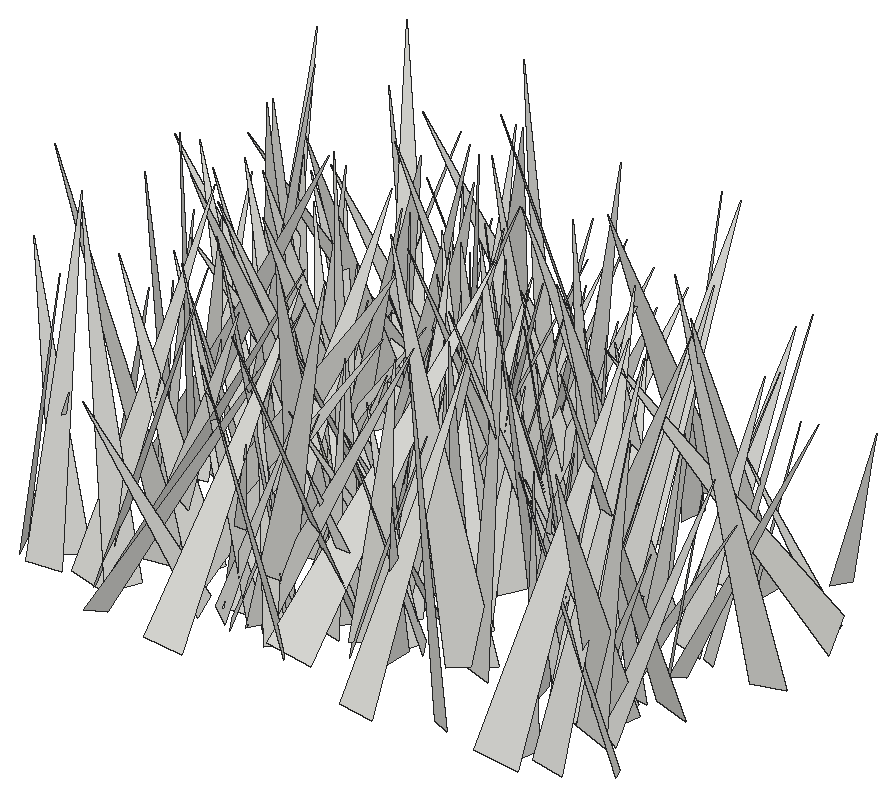
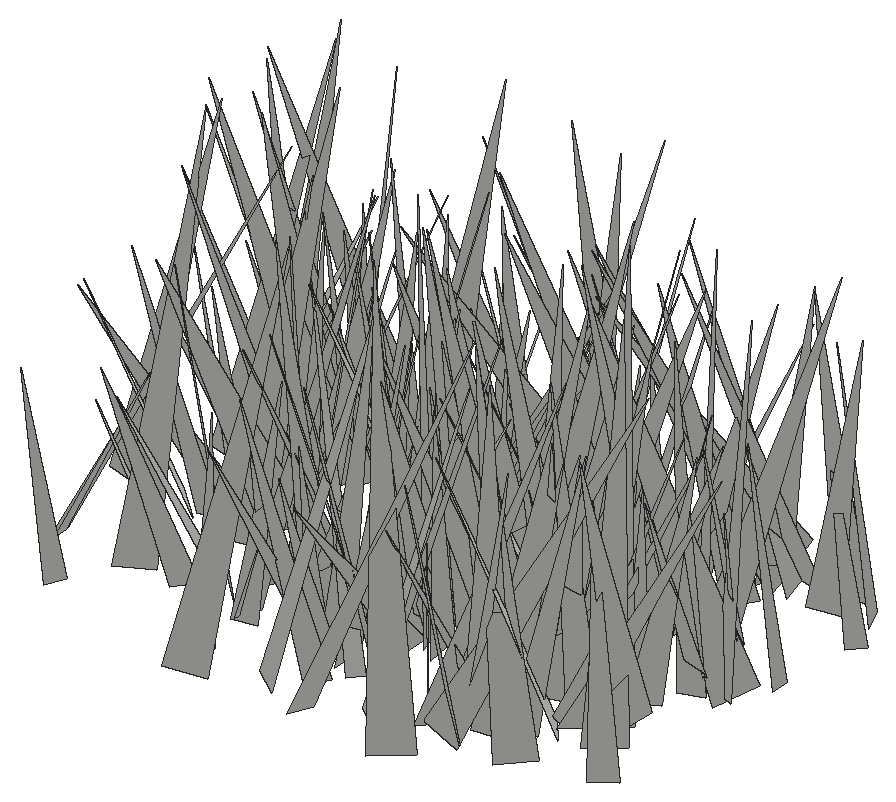
# SketchUp Ruby script. Lengths in inches.
U = 1.inch
M = Sketchup.active_model
def pt(a) = Geom::Point3d.new(a.map { |v| v * U })
def face(e, loops, mat)
  f = e.add_face(loops[0].map { |a| pt(a) })
  loops[1..].each { |l| e.add_face(l.map { |a| pt(a) }).erase! }
  f.material = f.back_material = mat if mat
  f
end
# faces: each face lists its corners as indices into pts; further lists are holes
def faces(e, pts, list, mat = nil) = list.each { |f| face(e, (f[0].is_a?(Array) ? f : [f]).map { |l| l.map { |i| pts[i] } }, mat) }
# xy, xz, yz: faces in a plane at the given z, y or x. An outline is a flat list of corners, or four numbers for a rectangle; further outlines are holes
def ring(l) = l.size == 4 ? [[l[0], l[1]], [l[2], l[1]], [l[2], l[3]], [l[0], l[3]]] : l.each_slice(2).to_a
def flat(e, list, mat, &to3) = list.each { |f| face(e, (f[0].is_a?(Array) ? f : [f]).map { |l| ring(l).map { |u, v| to3.(u, v) } }, mat) }
def xy(e, z, list, mat = nil) = flat(e, list, mat) { |x, y| [x, y, z] }
def xz(e, y, list, mat = nil) = flat(e, list, mat) { |x, z| [x, y, z] }
def yz(e, x, list, mat = nil) = flat(e, list, mat) { |y, z| [x, y, z] }
def lines(e, pts, list) = list.each { |a, b| e.add_line(pt(pts[a]), pt(pts[b])) }
# prism: a flat outline (further loops are holes) pulled along v
def prism(e, loops, v, mat = nil)
  f = face(e, loops, mat); d = Geom::Vector3d.new(v.map { |x| x * U })
  f.pushpull(f.normal.samedirection?(d) ? d.length : -d.length)
end
def box(e, o, s, mat = nil) = prism(e, [[o, [o[0] + s[0], o[1], o[2]], [o[0] + s[0], o[1] + s[1], o[2]], [o[0], o[1] + s[1], o[2]]]], [0, 0, s[2]], mat)
def at(x, y, z, deg = 0) = Geom::Transformation.translation(pt([x, y, z])) * Geom::Transformation.rotation(ORIGIN, Z_AXIS, deg.degrees)
def axes(o, x, y, z) = Geom::Transformation.new([*x, 0, *y, 0, *z, 0, *pt(o).to_a, 1])
def part(name) = M.definitions.add(name)
# library, detail: a bought-in or finely detailed component or shape, given as its bounding box
def library(name, o, s) = part(name).tap { |d| box(d.entities, o, s) }
def detail(e, o, s) = box(e.add_group.entities, o, s)
def put(e, d, t, mat = nil) = e.add_instance(d, t).tap { |i| i.material = mat if mat }
def group(e, t, mat = nil) = e.add_group.tap { |g| g.transformation = t; g.material = mat if mat }.entities
root = M.entities
c1 = part("fur_instance\#9")
p = [[0.8125,0,1.79],[0.67,-0.02,1.48],[0,-0.11,0],[0,0.11,0]]
faces(c1.entities,p,[[0,1,2,3]])
put(root,c1,axes([92.99,290.21,-27.1],[-4.59731,-1.23154,0.33008],[-1.08177,4.4213,1.42926],[0.67485,-1.30242,4.53973]))
put(root,c1,axes([96.88,289.59,-27.1],[-4.48858,-3.56813,1.07524],[-3.58767,4.5928,0.2643],[1.00813,0.45789,5.72792]))
put(root,c1,axes([104.22,288.76,-27.1],[-3.8782,-4.63911,2.52217],[-5.26639,3.62608,-1.42825],[0.38461,2.87286,5.87554]))
put(root,c1,axes([97.9375,292.27,-27.1],[-3.38776,-6.42257,0.32475],[-6.36234,3.40084,0.88702],[0.93573,-0.12917,7.20691]))
put(root,c1,axes([108.84,292.48,-27.1],[5.9537,-4.05045,0.58701],[-3.75603,-5.81897,-2.05648],[-1.62572,-1.38951,6.90098]))
put(root,c1,axes([93.57,287.27,-27.1],[-1.05391,6.67902,0.37292],[6.52998,1.10912,-1.41007],[1.4518,-0.14015,6.613]))
put(root,c1,axes([85.69,289.71,-27.1],[4.582,2.26461,1.64468],[2.3704,-4.81752,0.02956],[-1.48816,-0.70087,5.111]))
put(root,c1,axes([100.23,291.46,-27.1],[3.94789,-1.4658,0.35037],[-1.34081,-3.86465,-1.06014],[-0.68816,-0.87925,4.0756]))
put(root,c1,axes([101.4,287.75,-27.1],[0.40052,6.46259,0.29319],[6.45769,-0.38185,-0.40475],[0.38629,-0.31712,6.46233]))
put(root,c1,axes([95.36,290.65,-27.1],[6.75458,-3.1446,1.55563],[-3.25939,-6.87331,0.25842],[-1.29802,0.89549,7.44621]))
put(root,c1,axes([107.74,289.15,-27.1],[-4.70779,-0.34884,1.44292],[-0.70643,4.74641,-1.15738],[1.30563,1.3103,4.57662]))
put(root,c1,axes([89.0625,289.64,-27.1],[6.34041,1.92452,0.88463],[1.94009,-6.39712,0.01179],[-0.84995,-0.24555,6.62604]))
put(root,c1,axes([87.1,289,-27.1],[-0.4945,6.57851,1.5324],[6.75453,0.47319,0.14829],[-0.03697,-1.53911,6.5954]))
put(root,c1,axes([110.875,289.91,-27.1],[-4.67684,-2.75,0.36196],[-2.71074,4.38122,-1.73872],[-0.58771,1.67594,5.13928]))
put(root,c1,axes([107.12,288.09,-27.1],[-0.59068,7.87895,1.19707],[7.83923,0.79048,-1.33468],[1.43434,-1.07565,7.78752]))
put(root,c1,axes([90.06,289.53,-27.1],[-6.40273,2.01611,1.14645],[1.98655,6.50456,-0.34415],[1.19695,-0.01086,6.70383]))
put(root,c1,axes([90.33,287.71,-27.1],[6.45135,0.1489,0.38361],[-0.04006,-5.77049,2.9136],[-0.40954,2.91007,5.75787]))
put(root,c1,axes([95.1,290.56,-27.1],[5.1253,5.35023,0.94765],[5.22805,-4.50107,-2.86349],[1.48003,-2.62814,6.83331]))
put(root,c1,axes([93.77,290.09,-27.1],[2.51167,3.62255,0.80621],[3.69421,-2.34748,-0.96099],[0.35452,-1.20325,4.30208]))
put(root,c1,axes([87.31,290.25,-27.1],[1.60632,-4.77246,2.92285],[-5.28453,-2.29441,-0.84211],[-1.84207,2.42054,4.96463]))
put(root,c1,axes([84.92,291.53,-27.1],[1.46313,-3.34357,0.17988],[-3.25058,-1.37123,0.95187],[0.80348,0.54115,3.52337]))
put(root,c1,axes([108.59,291.33,-27.1],[1.5633,5.69815,3.01797],[6.40687,-1.02237,-1.38843],[0.72737,-3.24142,5.74326]))
put(root,c1,axes([94.44,289.79,-27.1],[3.52648,2.43175,0.31475],[2.41999,-3.54045,0.23962],[-0.3951,0.0194,4.27692]))
put(root,c1,axes([98.47,291.22,-27.1],[4.57096,2.53062,0.74602],[2.63797,-4.36083,-1.37058],[0.04077,-1.55993,5.04174]))
put(root,c1,axes([92.94,291.93,-27.1],[3.65052,-1.24636,0.3015],[-1.17659,-3.61738,-0.70767],[-0.50984,-0.576,3.79195]))
put(root,c1,axes([96.48,289.61,-27.1],[-4.58917,0.765,0.19448],[0.68534,4.43094,-1.25723],[0.3916,1.21042,4.47941]))
put(root,c1,axes([108.77,288.75,-27.1],[1.7832,7.11152,0.69499],[7.11724,-1.83129,0.47737],[-0.63379,-0.55606,7.31612]))
put(root,c1,axes([89.66,289.59,-27.1],[7.04502,0.38941,0.11832],[0.34745,-6.82295,1.76766],[-0.21195,1.75889,6.83077]))
put(root,c1,axes([94.96,290.58,-27.1],[-6.17227,-0.98801,0.5453],[-1.07692,6.06305,-1.2042],[0.3373,1.27815,6.13375]))
put(root,c1,axes([98.56,292.55,-27.1],[0.67909,-3.62862,0.46379],[-3.53581,-0.77205,-0.86319],[-0.93808,0.2832,3.58928]))
put(root,c1,axes([89.8,291.5625,-27.1],[3.48254,-4.50934,1.30252],[-4.66936,-3.1635,1.53235],[0.47726,1.95368,5.48763]))
put(root,c1,axes([98.82,291.65,-27.1],[3.55242,-4.27149,1.91187],[-4.60398,-3.6203,0.46613],[-0.83917,1.77997,5.53606]))
put(root,c1,axes([91.64,292.07,-27.1],[-5.50696,2.25656,1.40845],[2.52369,5.45565,1.12666],[0.84072,-1.59571,5.84374]))
put(root,c1,axes([88.83,289.13,-27.1],[1.55056,7.17303,0.47228],[7.18686,-1.53634,-0.26142],[0.15632,-0.51668,7.33405]))
put(root,c1,axes([96.16,291.125,-27.1],[-6.23091,-2.8217,1.23434],[-3.03851,6.08694,-1.42355],[0.50305,1.81577,6.69027]))
put(root,c1,axes([100.48,292.57,-27.1],[-3.61255,-2.36918,0.54232],[-2.35627,3.65218,0.25916],[0.59592,0.07847,4.31235]))
put(root,c1,axes([102.52,292.57,-27.1],[2.49125,-7.31611,3.2771],[-7.62751,-3.2193,-1.38865],[-2.46697,2.5655,7.60286]))
put(root,c1,axes([97.47,291.28,-27.1],[1.36793,4.62634,1.5435],[4.80198,-1.5578,0.41343],[-0.85231,-1.35162,4.8066]))
put(root,c1,axes([91.45,291.71,-27.1],[4.41498,5.25807,0.18984],[4.81628,-3.93899,-2.90917],[2.11822,-2.00311,6.21901]))
put(root,c1,axes([109.58,294.375,-27.1],[-2.16653,-7.31637,0.90738],[-7.36569,2.18851,0.05952],[0.3151,0.85299,7.63018]))
put(root,c1,axes([107.79,292.02,-27.1],[3.74369,-0.67268,0.40161],[-0.71907,-3.7286,0.45768],[-0.31101,0.52348,3.776]))
put(root,c1,axes([104.64,292.85,-27.1],[4.0424,-1.6774,0.68877],[-1.67315,-4.09915,-0.16314],[-0.69903,0.11126,4.37357]))
put(root,c1,axes([89.69,292.63,-27.1],[-2.64388,-6.79077,2.11498],[-6.99476,2.07362,-2.08599],[-1.28885,2.67645,6.98236]))
put(root,c1,axes([100.11,292.27,-27.1],[-4.10178,1.61092,0.95507],[1.70987,4.15942,0.32775],[0.76391,-0.66031,4.39457]))
put(root,c1,axes([104.35,294.11,-27.1],[-6.11732,-3.75265,2.76683],[-3.28898,6.70851,1.82699],[3.3046,-0.26993,6.94018]))
put(root,c1,axes([108.62,293.43,-27.1],[-4.68733,-0.90911,0.30449],[-0.85582,4.65242,0.7161],[0.43216,-0.64711,4.72067]))
put(root,c1,axes([105.49,292.61,-27.1],[4.4988,1.24272,1.44893],[1.33102,-4.70119,-0.10058],[-1.36826,-0.48722,4.6662]))
put(root,c1,axes([107.02,291.88,-27.1],[0.33091,4.05955,1.18914],[3.81261,-0.80293,1.68011],[-1.83248,-0.93747,3.71034]))
put(root,c1,axes([109.0625,291.67,-27.1],[2.45412,4.72767,0.6627],[4.74881,-2.3413,-0.8831],[0.48874,-0.99004,5.25297]))
put(root,c1,axes([93.49,295.4,-27.1],[6.57894,-4.30915,0.69378],[-4.10201,-6.53322,-1.6802],[-1.49116,-1.03963,7.68298]))
put(root,c1,axes([98.35,294.93,-27.1],[-4.30266,-2.43803,0.04686],[-2.30354,4.09498,1.544],[0.79994,-1.32144,4.69819]))
put(root,c1,axes([97.22,289.41,-27.1],[-2.37553,7.32496,0.20013],[6.77476,2.27563,-2.87444],[2.79244,0.71043,7.14393]))
put(root,c1,axes([99.4,294.49,-27.1],[-2.79932,-5.24784,0.26282],[-5.09915,2.64134,-1.57068],[-1.26789,0.96362,5.73663]))
put(root,c1,axes([90.03,293.66,-27.1],[5.30447,3.34271,0.68413],[3.37643,-4.96043,-1.94241],[0.49141,-1.99988,5.96139]))
put(root,c1,axes([90.14,294.2,-27.1],[3.5795,-7.50714,1.0436],[-6.77337,-2.6505,4.166],[3.40115,2.62237,7.19823]))
put(root,c1,axes([98,294.3,-27.1],[3.54062,0.10617,1.20258],[0.38468,-3.63127,-0.812],[-1.14433,-0.89222,3.44788]))
put(root,c1,axes([107.23,291.7,-27.1],[6.03648,4.13261,1.07509],[4.02235,-6.12795,0.97074],[-1.43354,0.20766,7.25088]))
put(root,c1,axes([105.37,294.56,-27.1],[4.87258,-2.82126,2.84071],[-2.53321,-5.63755,-1.25383],[-3.10033,0.17232,5.48903]))
put(root,c1,axes([94.46,290.65,-27.1],[-4.73234,6.09922,1.47861],[5.53404,4.92888,-2.61961],[2.95993,0.53615,7.26177]))
put(root,c1,axes([103.02,292.25,-27.1],[2.9733,6.47594,2.08154],[6.51847,-3.36189,1.14821],[-1.94427,-1.36785,7.03277]))
put(root,c1,axes([107.44,291.62,-27.1],[-5.06165,5.7028,1.49455],[5.55918,5.27278,-1.292],[1.96243,-0.22764,7.51486]))
put(root,c1,axes([95.7,295.18,-27.1],[-1.12897,-3.54048,0.33773],[-3.515,1.16474,0.46018],[0.54205,0.17891,3.68752]))
put(root,c1,axes([105.26,293.57,-27.1],[6.69732,-3.52244,1.21858],[-3.71872,-6.48437,1.69431],[-0.25228,2.07171,7.37503]))
put(root,c1,axes([105.63,295.02,-27.1],[-6.50715,-2.26194,0.29712],[-2.26712,6.51165,-0.07913],[0.25462,0.17236,6.88863]))
put(root,c1,axes([99.84,295.36,-27.1],[-1.49561,-5.63035,1.67127],[-5.71638,1.79132,0.91926],[1.34798,1.34949,5.75262]))
put(root,c1,axes([102,293.28,-27.1],[-0.34341,4.80516,0.97397],[4.88667,0.41477,-0.32328],[0.39826,-0.94579,4.80656]))
put(root,c1,axes([88.99,294.71,-27.1],[-4.49865,-5.44108,2.87885],[-5.83326,4.90701,0.15896],[1.96626,2.10876,7.05818]))
put(root,c1,axes([99.17,295.5,-27.1],[-0.33006,-3.76044,0.39687],[-3.50265,0.15395,-1.45434],[-1.42474,0.49269,3.4835]))
put(root,c1,axes([105.125,295,-27.1],[-5.04486,-3.51647,1.75014],[-3.733,5.17856,-0.35556],[1.22196,1.30239,6.1392]))
put(root,c1,axes([97.53,292.36,-27.1],[-7.91635,-0.39433,1.24518],[-0.80795,7.48837,-2.76517],[1.02625,2.85367,7.42819]))
put(root,c1,axes([95.72,295.375,-27.1],[2.4486,-4.30122,0.69777],[-4.269,-2.2075,1.37318],[0.8735,1.26866,4.75506]))
put(root,c1,axes([108.26,294.24,-27.1],[1.91991,5.69676,2.84026],[5.7974,-2.78995,1.67703],[-2.62873,-1.9923,5.77292]))
put(root,c1,axes([85.29,295.17,-27.1],[4.21688,0.53755,0.91963],[0.65776,-4.26755,-0.52159],[-0.83787,-0.64478,4.21888]))
put(root,c1,axes([94.41,294.0625,-27.1],[3.13129,2.44329,0.37399],[2.42945,-3.15346,0.26073],[-0.45532,-0.0231,3.96316]))
put(root,c1,axes([97.3,295.13,-27.1],[-3.1283,2.85302,0.75954],[2.94685,2.94951,1.058],[-0.18092,-1.28978,4.09959]))
put(root,c1,axes([108.72,295.12,-27.1],[3.70099,1.78589,1.07617],[1.91017,-3.78303,-0.29128],[-0.83593,-0.7377,4.09901]))
put(root,c1,axes([93.85,295.02,-27.1],[3.11489,-2.67244,0.85057],[-2.80172,-2.90834,1.1224],[0.12545,1.40269,3.94774]))
put(root,c1,axes([88.76,293.07,-27.1],[2.37609,4.94692,0.8109],[4.47755,-2.49789,2.11838],[-2.25414,0.25283,5.06264]))
put(root,c1,axes([90.92,294.7,-27.1],[-2.13288,4.47426,0.69403],[4.36785,1.83113,1.61826],[-1.19274,-1.2953,4.68502]))
put(root,c1,axes([98.67,293.7,-27.1],[-5.11212,3.73872,1.49873],[3.53116,5.32488,-1.23875],[1.93782,0.15985,6.21106]))
put(root,c1,axes([86.32,296.91,-27.1],[-2.86307,-5.78602,1.82095],[-5.78172,3.21211,1.11581],[1.83453,1.09334,6.35847]))
put(root,c1,axes([89.88,296.82,-27.1],[-3.92886,-2.51502,0.86647],[-2.44083,4.02285,0.60923],[1.05758,-0.05874,4.62495]))
put(root,c1,axes([93.2,298.875,-27.1],[6.13444,-4.45258,1.42838],[-3.84619,-6.14459,-2.6359],[-2.65943,-1.38408,7.10696]))
put(root,c1,axes([107.1875,295.24,-27.1],[3.6219,-1.04912,0.12415],[-1.02885,-3.40219,1.26523],[0.23987,1.24847,3.55218]))
put(root,c1,axes([98.68,293.49,-27.1],[6.48387,0.57283,2.72889],[-0.5216,-6.53637,2.61139],[-2.73914,2.60063,5.96233]))
put(root,c1,axes([105.375,298.73,-27.1],[3.52334,-7.25518,1.10129],[-7.15699,-3.66725,-1.26216],[-1.62106,0.42196,7.96608]))
put(root,c1,axes([86.93,295.41,-27.1],[1.67627,3.15128,1.04901],[3.10636,-1.90337,0.75402],[-1.17538,-0.53615,3.48882]))
put(root,c1,axes([93.32,298.4,-27.1],[-6.61379,-2.13915,0.88077],[-1.88588,6.53057,1.69974],[1.33985,-1.36736,6.74011]))
put(root,c1,axes([87.22,297.46,-27.1],[-0.17668,-5.97479,1.5156],[-5.97573,0.53792,1.42395],[1.51188,1.4279,5.80532]))
put(root,c1,axes([91.88,298.78,-27.1],[0.79588,-7.21699,0.96951],[-7.03929,-1.01213,-1.75565],[-1.86367,0.74092,7.04528]))
put(root,c1,axes([86,296.6,-27.1],[7.56022,-3.29271,0.03526],[-3.23696,-7.41517,1.59297],[0.60437,1.47429,8.09082]))
put(root,c1,axes([101.08,294.47,-27.1],[-1.83761,6.5724,0.07775],[6.30696,1.74042,1.94227],[-1.85059,-0.59481,6.54223]))
put(root,c1,axes([94.9,295.95,-27.1],[-3.18645,2.79123,0.05753],[2.78151,3.16651,0.42911],[-0.23972,-0.36053,4.21429]))
put(root,c1,axes([106.25,294.69,-27.1],[1.83288,7.01444,0.75411],[7.05484,-1.82448,-0.17632],[-0.01908,-0.77421,7.24781]))
put(root,c1,axes([90.8,297.09,-27.1],[4.14208,3.82367,0.06036],[3.46383,-3.71363,-2.44781],[1.62049,-1.8356,5.07794]))
put(root,c1,axes([111.08,297.66,-27.1],[-1.04276,-7.37455,2.60053],[-7.71345,0.53914,-1.56404],[-1.28435,2.74945,7.28184]))
put(root,c1,axes([100.48,297.59,-27.1],[-5.43342,3.18473,2.47254],[3.60205,5.6984,0.57576],[1.81141,-1.77869,6.27161]))
put(root,c1,axes([92.75,297.48,-27.1],[6.6153,-1.38256,1.33275],[-1.44359,-6.733,0.18083],[-1.26639,0.45296,6.75581]))
put(root,c1,axes([98.95,300.47,-27.1],[-6.12859,-4.53414,1.24355],[-3.97845,6.08997,2.59781],[2.50535,-1.42065,7.16724]))
put(root,c1,axes([98.54,298.05,-27.1],[5.36268,3.16176,1.79895],[3.56295,-5.21159,-1.4615],[-0.73371,-2.1986,6.05138]))
put(root,c1,axes([90.08,295.65,-27.1],[-7.4216,0.05563,3.73189],[-0.80703,8.0859,-1.72548],[3.64401,1.90407,7.21845]))
put(root,c1,axes([106.25,297.29,-27.1],[4.13039,-0.87619,1.21239],[-0.99071,-4.26996,0.28929],[-1.12075,0.54542,4.21238]))
put(root,c1,axes([103.47,297.64,-27.1],[-3.24328,-4.06122,2.56752],[-4.33534,3.80899,0.54855],[2.07134,1.61325,5.16831]))
put(root,c1,axes([99.17,297.72,-27.1],[-0.52973,-5.32119,2.08202],[-5.65742,0.19488,-0.94137],[-0.8022,2.1395,5.26399]))
put(root,c1,axes([99.83,296.15,-27.1],[4.69636,2.95892,0.9191],[2.85112,-4.78039,0.82137],[-1.21287,0.21986,5.48965]))
put(root,c1,axes([91.32,297.74,-27.1],[-4.7653,3.97573,1.88545],[4.327,4.73874,0.94381],[0.79899,-1.95123,6.13381]))
put(root,c1,axes([95.32,295.34,-27.1],[3.44077,4.42208,0.21812],[4.18127,-3.33634,1.68138],[-1.45578,0.8691,5.34478]))
put(root,c1,axes([93.6,296.52,-27.1],[-4.4668,1.24969,0.75909],[0.98308,4.37301,-1.41442],[1.08236,1.18546,4.4174]))
put(root,c1,axes([110.65,301.82,-27.1],[-7.29463,-2.71144,0.02018],[-2.47986,6.69465,3.09773],[1.09665,-2.89718,7.13916]))
put(root,c1,axes([108.3,296.3,-27.1],[5.03908,0.51167,0.65236],[0.18588,-4.61324,2.18248],[-0.80798,2.12978,4.57066]))
put(root,c1,axes([96.32,298.16,-27.1],[-1.6675,3.7386,1.84502],[3.94069,2.06209,-0.61692],[1.36097,-1.39013,4.04687]))
put(root,c1,axes([98.68,298.3,-27.1],[-3.99392,-3.16377,0.39905],[-3.06383,3.62986,-1.88605],[-0.88412,1.71311,4.73326]))
put(root,c1,axes([90.98,298.25,-27.1],[-5.83458,-0.97839,0.23219],[-1.00024,5.78729,-0.74851],[0.10327,0.77686,5.8685]))
put(root,c1,axes([95.36,297.41,-27.1],[2.13777,3.57515,0.4757],[3.58502,-2.16686,0.17428],[-0.39447,-0.3179,4.1619]))
put(root,c1,axes([97.27,299.82,-27.1],[3.86717,-5.0611,1.49434],[-5.13106,-4.03908,-0.40116],[-1.23289,0.93486,6.35679]))
put(root,c1,axes([94.0625,298.15,-27.1],[7.6269,-0.50277,1.8471],[-0.68475,-7.80192,0.70374],[-1.78765,0.84341,7.61099]))
put(root,c1,axes([91.01,300.65,-27.1],[4.14575,-5.15062,1.64406],[-4.88287,-4.45639,-1.64839],[-2.32151,0.17524,6.40304]))
put(root,c1,axes([87.81,300.9,-27.1],[7.83218,-2.47016,1.5817],[-2.12062,-7.88445,-1.81244],[-2.02643,-1.29626,8.00998]))
put(root,c1,axes([96.875,299.8,-27.1],[6.48852,0.93317,0.66882],[1.0636,-6.33108,-1.48501],[-0.43231,-1.57025,6.38486]))
put(root,c1,axes([107.39,297.95,-27.1],[0.7475,5.23214,1.319],[5.34274,-0.53135,-0.92008],[0.75507,-1.41992,5.20456]))
put(root,c1,axes([96.4,297.22,-27.1],[-5.56085,2.56326,1.5764],[2.25423,5.74256,-1.38556],[1.99343,0.65656,5.96435]))
put(root,c1,axes([89.48,297.54,-27.1],[-0.14147,5.00237,0.6936],[4.87308,-0.04695,1.33257],[-1.32587,-0.70632,4.82369]))
put(root,c1,axes([96.59,297.81,-27.1],[5.74165,3.30721,0.02247],[3.30582,-5.73764,-0.2359],[0.09829,-0.21562,6.62182]))
put(root,c1,axes([87.33,296.8,-27.1],[0.66443,5.27954,0.01832],[5.19176,-0.65673,0.9642],[-0.95891,0.10252,5.2331]))
put(root,c1,axes([96.35,299.97,-27.1],[7.03768,2.72348,2.80411],[3.28727,-7.24831,-1.21043],[-2.11523,-2.20318,7.44856]))
put(root,c1,axes([107.13,302.28,-27.1],[6.98894,-3.62557,1.01436],[-3.15649,-6.80873,-2.58782],[-2.05189,-1.87497,7.43594]))
put(root,c1,axes([89.54,301.65,-27.1],[-5.28354,-0.86585,0.73138],[-0.45173,4.80676,2.42722],[1.0395,-2.31209,4.77222]))
put(root,c1,axes([102.47,299.21,-27.1],[-6.58404,0.20466,2.39247],[0.20033,7.00521,-0.04793],[2.39284,-0.02336,6.58705]))
put(root,c1,axes([88.05,298.98,-27.1],[-4.17135,3.80631,1.04328],[3.93898,4.10999,0.75433],[0.24669,-1.26356,5.59635]))
put(root,c1,axes([93.47,300.63,-27.1],[6.15872,-4.73604,0.69713],[-4.78091,-6.14284,0.50431],[-0.2428,0.82545,7.75278]))
put(root,c1,axes([92.97,297.76,-27.1],[0.07199,5.81915,0.58708],[5.58747,-0.24194,1.7129],[-1.72841,-0.53974,5.5618]))
put(root,c1,axes([90.65,299.52,-27.1],[2.6007,2.51832,0.88377],[2.64819,-2.58836,-0.41733],[-0.33183,-0.9193,3.59603]))
put(root,c1,axes([94.6,298.76,-27.1],[-4.83197,-1.5354,1.95575],[-2.0901,4.8234,-1.3772],[1.34681,1.9768,4.87942]))
put(root,c1,axes([102.23,302.35,-27.1],[-7.41474,-1.37074,2.09218],[-0.74138,7.45582,2.25736],[2.38883,-1.94072,7.19456]))
put(root,c1,axes([89.79,300.04,-27.1],[5.47744,-1.647,1.93505],[-1.81976,-5.75174,0.25556],[-1.77356,0.81501,5.71398]))
put(root,c1,axes([91.16,299.27,-27.1],[-3.95377,2.90545,0.68572],[2.92437,3.99824,-0.07937],[0.59996,-0.34142,4.90588]))
put(root,c1,axes([98.46,302.09,-27.1],[-3.60567,-4.25836,0.82426],[-4.10665,3.69659,1.13335],[1.39586,-0.12438,5.46351]))
put(root,c1,axes([98.72,300.18,-27.1],[3.89411,3.28531,3.07479],[3.51498,-4.75969,0.63397],[-2.80935,-1.40135,5.05524]))
put(root,c1,axes([87.25,302.03,-27.1],[5.45655,-4.97036,1.37233],[-4.9464,-5.60993,-0.6508],[-1.45634,0.43117,7.35221]))
put(root,c1,axes([108.48,297.73,-27.1],[3.77258,4.9169,0.38845],[4.64704,-3.70729,1.79444],[-1.65279,0.7995,5.93196]))
put(root,c1,axes([93.42,299.4,-27.1],[6.3266,0.04535,0.7535],[-0.10627,-6.24313,1.26797],[-0.74735,1.27161,6.1984]))
put(root,c1,axes([104.79,296.97,-27.1],[-5.35866,5.61511,0.59327],[5.12673,5.1813,-2.73266],[2.36603,1.4904,7.2648]))
put(root,c1,axes([90.61,303.77,-27.1],[1.9178,-7.47283,0.23219],[-7.45531,-1.92947,-0.52008],[-0.56157,0.09505,7.69744]))
put(root,c1,axes([96.58,299.13,-27.1],[-2.91269,3.59929,0.76549],[3.33369,2.99435,-1.39463],[1.55801,0.3218,4.41516]))
put(root,c1,axes([88.9,301.68,-27.1],[-5.72955,1.74546,0.28048],[1.75274,5.48455,1.67353],[-0.23061,-1.68113,5.75097]))
put(root,c1,axes([110.54,301.98,-27.1],[-3.53813,-0.73541,0.01575],[-0.72603,3.50386,0.50526],[0.11809,-0.49152,3.57826]))
put(root,c1,axes([96.75,303.4375,-27.1],[6.70588,0.95076,0.50826],[1.07552,-6.12086,-2.74035],[-0.07444,-2.78609,6.19381]))
put(root,c1,axes([100.63,301.4,-27.1],[-4.67838,0.58429,0.4377],[0.60816,4.68963,0.24018],[0.40387,-0.29353,4.7086]))
put(root,c1,axes([95.62,300.23,-27.1],[-5.53054,0.45224,1.5037],[0.10523,5.59989,-1.29715],[1.5667,1.22031,5.39525]))
put(root,c1,axes([108.17,299.96,-27.1],[2.52886,2.74781,0.4271],[2.47453,-2.48701,1.34889],[-1.2687,0.62635,3.48225]))
put(root,c1,axes([98.375,300.44,-27.1],[2.55836,5.15566,0.46861],[5.11042,-2.43162,-1.14739],[0.82709,-0.92305,5.63999]))
put(root,c1,axes([102.81,300.17,-27.1],[-3.06168,2.49465,0.02952],[2.42804,2.99025,-0.87237],[0.57338,0.65813,3.85176]))
put(root,c1,axes([97.04,298.8,-27.1],[-6.53703,2.92768,0.70077],[2.53956,6.26275,-2.47462],[1.61648,2.00045,6.72163]))
put(root,c1,axes([99.73,301.51,-27.1],[6.98669,-0.82296,2.45735],[-1.02769,-7.36659,0.45485],[-2.37901,0.76535,7.02027]))
put(root,c1,axes([101.95,302.88,-27.1],[1.41164,-4.04262,0.99191],[-4.10193,-1.52908,-0.39425],[-0.70768,0.79907,4.26381]))
put(root,c1,axes([92.08,304.8,-27.1],[-0.45254,-7.13046,0.09555],[-6.72101,0.39447,-2.39372],[-2.38342,0.24148,6.7319]))
put(root,c1,axes([89.96,303.11,-27.1],[3.58153,-3.37168,2.12142],[-3.21603,-4.13077,-1.13573],[-2.3507,0.51427,4.78599]))
put(root,c1,axes([92.88,304.55,-27.1],[-6.34287,-0.8603,1.40577],[-0.30586,6.10717,2.3574],[1.61949,-2.21602,5.95103]))
put(root,c1,axes([95.55,303.83,-27.1],[-6.52757,-2.25287,1.08541],[-2.07972,6.57544,1.14066],[1.38863,-0.74224,6.81054]))
put(root,c1,axes([105.32,300.46,-27.1],[3.38702,2.66566,0.2184],[2.51461,-3.29384,1.20529],[-0.91115,0.81867,4.13823]))
put(root,c1,axes([96.9375,301.99,-27.1],[4.58071,3.98416,0.78034],[4.05613,-4.44078,-1.1369],[0.17387,-1.36793,5.96354]))
put(root,c1,axes([97.68,302.71,-27.1],[-6.3571,-0.05635,1.63328],[-0.03082,6.56286,0.10646],[1.63396,-0.09544,6.35645]))
put(root,c1,axes([99.87,301.62,-27.1],[-4.04138,0.55951,1.25439],[0.25517,4.13619,-1.02282],[1.34961,0.89343,3.94964]))
put(root,c1,axes([103.8,301.34,-27.1],[4.42049,5.15695,1.86392],[5.12768,-4.73588,0.94203],[-1.94301,-0.76574,6.72662]))
put(root,c1,axes([87.53,300.21,-27.1],[-6.45449,2.84921,1.13675],[2.42101,6.35763,-2.18855],[1.88385,1.59157,6.70736]))
put(root,c1,axes([88.92,304.7,-27.1],[3.49272,-6.19271,0.17705],[-6.11252,-3.41157,1.25629],[1.00898,0.76914,6.99789]))
put(root,c1,axes([85.82,303.89,-27.1],[2.40691,-4.24835,1.2679],[-4.42272,-2.4014,0.34948],[-0.30924,1.27831,4.87028]))
put(root,c1,axes([98.8125,301.83,-27.1],[1.70019,7.5386,2.42367],[7.33263,-2.43467,2.42902],[-2.9895,-1.68439,7.33628]))
put(root,c1,axes([96.51,300.68,-27.1],[-3.43381,3.18637,0.41007],[2.54254,3.06224,-2.50406],[1.96382,1.60682,3.959]))
put(root,c1,axes([98.88,305.58,-27.1],[-4.98525,-6.36904,1.05647],[-6.36247,5.07321,0.56124],[1.09531,0.48105,8.06861]))
put(root,c1,axes([94.84,305.27,-27.1],[-4.07639,-4.57708,0.71562],[-4.52519,4.13816,0.69067],[0.99219,0.06853,6.09012]))
put(root,c1,axes([96.23,302.93,-27.1],[3.37327,4.28522,1.21914],[4.44713,-3.33099,-0.5966],[-0.2692,-1.33033,5.4209]))
put(root,c1,axes([105.11,302.125,-27.1],[-1.9043,4.31856,1.08738],[4.14528,2.15112,-1.28374],[1.62757,-0.42591,4.54184]))
put(root,c1,axes([98.31,303.05,-27.1],[-2.24113,2.46388,1.48853],[2.36542,2.65133,-0.82724],[1.6405,-0.45695,3.22631]))
put(root,c1,axes([101.4,306.77,-27.1],[2.31085,-7.14722,0.11909],[-7.10013,-2.30949,-0.83147],[-0.82765,-0.14321,7.46535]))
put(root,c1,axes([89.24,302.06,-27.1],[4.55508,3.875,0.43107],[3.83788,-4.57312,0.55448],[-0.68713,0.14532,5.95457]))
put(root,c1,axes([94.1,302.9375,-27.1],[2.37526,2.53476,1.46683],[2.25858,-2.78775,1.16004],[-1.86424,-0.14786,3.27432]))
put(root,c1,axes([91.24,302.94,-27.1],[1.22352,3.80068,0.33063],[3.61313,-1.04295,-1.38167],[1.22465,-0.72012,3.74608]))
put(root,c1,axes([101.875,305.17,-27.1],[3.65469,-1.69105,0.3912],[-1.57801,-3.61693,-0.89287],[-0.72291,-0.65395,3.92673]))
put(root,c1,axes([97.49,304.55,-27.1],[1.64693,-4.65446,0.85777],[-4.4282,-1.19483,2.01879],[1.67056,1.42146,4.50564]))
put(root,c1,axes([91.71,302.74,-27.1],[-3.76745,6.43232,1.47995],[6.58457,3.78058,0.33053],[0.45645,-1.44608,7.44709]))
put(root,c1,axes([108.6,304.66,-27.1],[3.31097,-1.72543,0.32906],[-1.73993,-3.31791,0.10944],[-0.24091,0.24944,3.73197]))
put(root,c1,axes([92.49,306.88,-27.1],[2.66865,-7.95792,0.14871],[-7.80747,-2.5868,1.68053],[1.54726,0.67254,8.22351]))
put(root,c1,axes([92.2,302.93,-27.1],[-6.19983,-0.76734,1.02255],[-1.02443,6.01091,-1.70052],[0.76483,1.83095,6.01123]))
put(root,c1,axes([98.97,302.61,-27.1],[-0.26739,4.57604,0.32256],[4.40279,0.34673,-1.26925],[1.2883,-0.2352,4.40462]))
put(root,c1,axes([96.78,306.39,-27.1],[-7.42366,-0.80204,0.92134],[-0.52005,7.2098,2.08597],[1.1053,-1.9946,7.16957]))
put(root,c1,axes([91.37,304.74,-27.1],[3.19088,3.17646,1.19509],[3.39239,-3.03309,-0.99593],[-0.09903,-1.55252,4.39087]))
